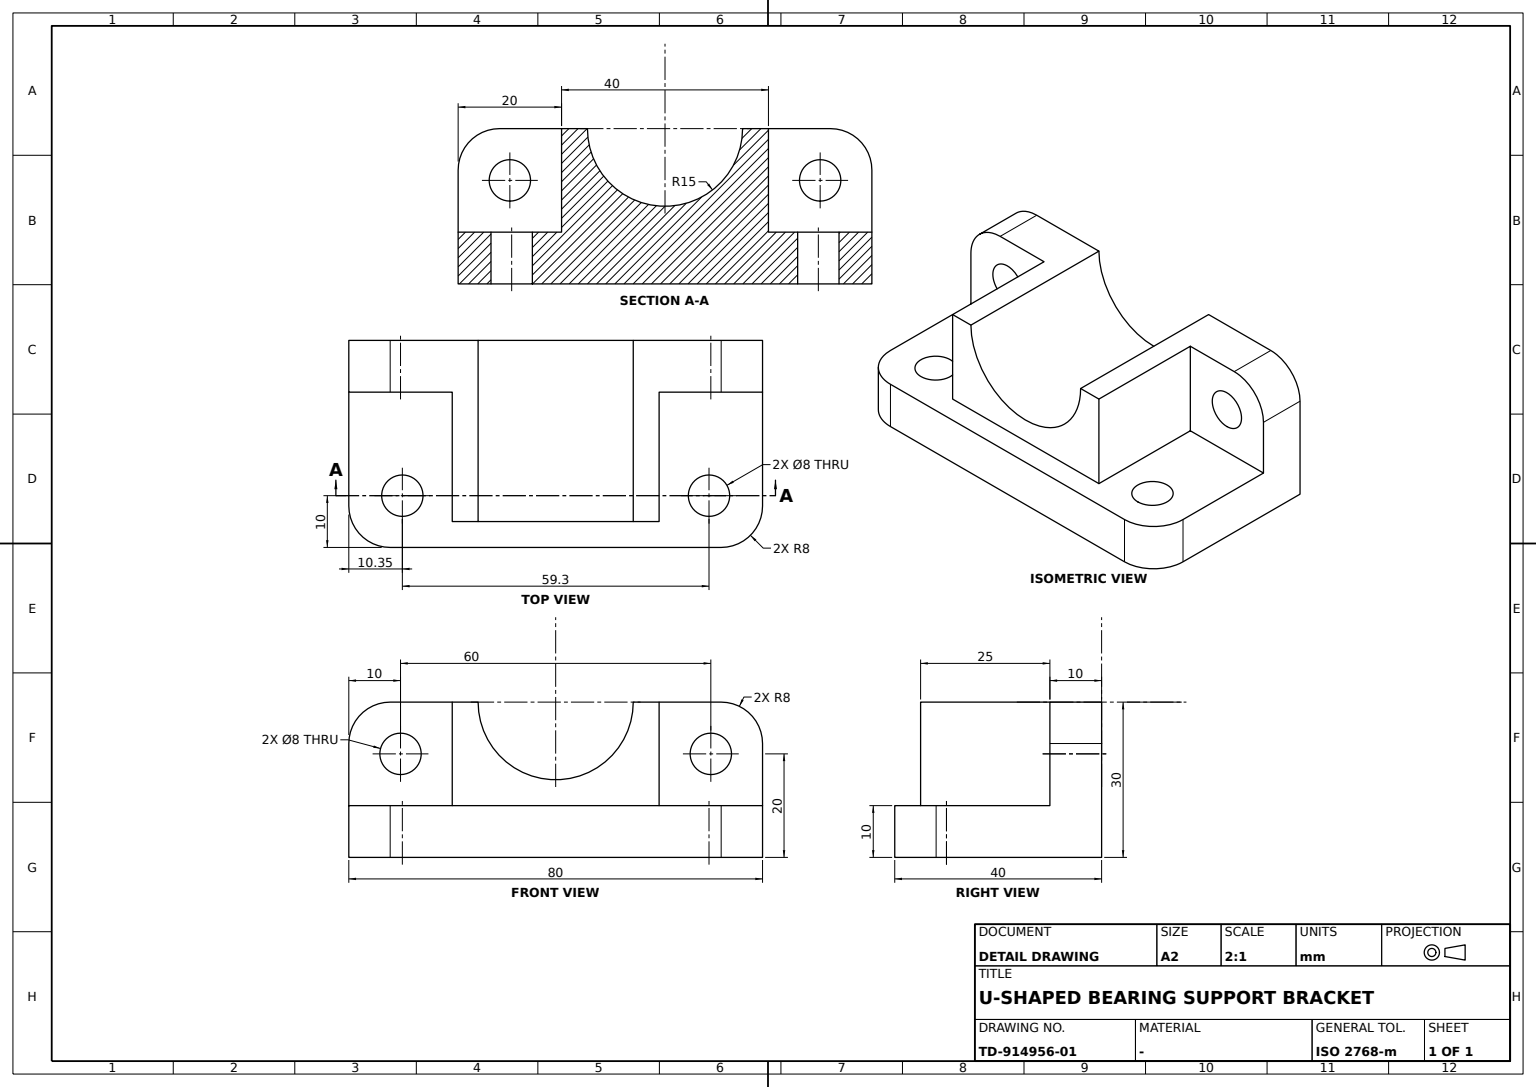
ISO-10303-21;
HEADER;
FILE_DESCRIPTION((''),'2;1');
FILE_NAME('','',(''),(''),'','','');
FILE_SCHEMA(('AUTOMOTIVE_DESIGN'));
ENDSEC;
DATA;
#1=APPLICATION_CONTEXT('');
#2=PRODUCT_CONTEXT('',#1,'mechanical');
#3=PRODUCT('','','',(#2));
#4=PRODUCT_DEFINITION_FORMATION('','',#3);
#5=PRODUCT_DEFINITION_CONTEXT('',#1,'design');
#6=PRODUCT_DEFINITION('','',#4,#5);
#7=PRODUCT_DEFINITION_SHAPE('','',#6);
#8=(LENGTH_UNIT()NAMED_UNIT(*)SI_UNIT(.MILLI.,.METRE.));
#9=(NAMED_UNIT(*)PLANE_ANGLE_UNIT()SI_UNIT($,.RADIAN.));
#10=(NAMED_UNIT(*)SI_UNIT($,.STERADIAN.)SOLID_ANGLE_UNIT());
#11=UNCERTAINTY_MEASURE_WITH_UNIT(LENGTH_MEASURE(0.005),#8,'distance_accuracy_value','');
#12=(GEOMETRIC_REPRESENTATION_CONTEXT(3)GLOBAL_UNCERTAINTY_ASSIGNED_CONTEXT((#11))GLOBAL_UNIT_ASSIGNED_CONTEXT((#8,#9,#10))REPRESENTATION_CONTEXT('',''));
#13=CARTESIAN_POINT('',(32.,-40.,-5.));
#14=VERTEX_POINT('',#13);
#15=CARTESIAN_POINT('',(32.,-40.,-15.));
#16=VERTEX_POINT('',#15);
#17=CARTESIAN_POINT('',(32.,-40.,-4.));
#18=DIRECTION('',(0.,0.,-1.));
#19=VECTOR('',#18,1000.);
#20=LINE('',#17,#19);
#21=EDGE_CURVE('',#14,#16,#20,.T.);
#22=ORIENTED_EDGE('',*,*,#21,.F.);
#23=CARTESIAN_POINT('',(10.,-40.,-5.));
#24=VERTEX_POINT('',#23);
#25=CARTESIAN_POINT('',(0.,-40.,-5.));
#26=DIRECTION('',(1.,0.,0.));
#27=VECTOR('',#26,1000.);
#28=LINE('',#25,#27);
#29=EDGE_CURVE('',#24,#14,#28,.T.);
#30=ORIENTED_EDGE('',*,*,#29,.F.);
#31=CARTESIAN_POINT('',(10.,-40.,7.));
#32=VERTEX_POINT('',#31);
#33=CARTESIAN_POINT('',(10.,-40.,0.));
#34=DIRECTION('',(0.,0.,1.));
#35=VECTOR('',#34,1000.);
#36=LINE('',#33,#35);
#37=EDGE_CURVE('',#24,#32,#36,.T.);
#38=ORIENTED_EDGE('',*,*,#37,.T.);
#39=CARTESIAN_POINT('',(0.,-40.,7.));
#40=VERTEX_POINT('',#39);
#41=CARTESIAN_POINT('',(5.,-40.,7.));
#42=LINE('',#41,#27);
#43=EDGE_CURVE('',#40,#32,#42,.T.);
#44=ORIENTED_EDGE('',*,*,#43,.F.);
#45=CARTESIAN_POINT('',(0.,-40.,-15.));
#46=VERTEX_POINT('',#45);
#47=CARTESIAN_POINT('',(0.,-40.,0.));
#48=LINE('',#47,#35);
#49=EDGE_CURVE('',#46,#40,#48,.T.);
#50=ORIENTED_EDGE('',*,*,#49,.F.);
#51=LINE('',#45,#27);
#52=EDGE_CURVE('',#46,#16,#51,.T.);
#53=ORIENTED_EDGE('',*,*,#52,.T.);
#54=EDGE_LOOP('',(#22,#30,#38,#44,#50,#53));
#55=FACE_BOUND('',#54,.T.);
#56=DIRECTION('',(0.,1.,0.));
#57=AXIS2_PLACEMENT_3D('',#45,#56,#34);
#58=PLANE('',#57);
#59=ADVANCED_FACE('',(#55),#58,.F.);
#60=CARTESIAN_POINT('',(0.,30.,1.));
#61=VERTEX_POINT('',#60);
#62=CARTESIAN_POINT('',(0.,30.,5.));
#63=AXIS2_PLACEMENT_3D('',#62,#26,#18);
#64=CIRCLE('',#63,4.);
#65=EDGE_CURVE('',#61,#61,#64,.T.);
#66=ORIENTED_EDGE('',*,*,#65,.T.);
#67=EDGE_LOOP('',(#66));
#68=FACE_BOUND('',#67,.T.);
#69=CARTESIAN_POINT('',(0.,-30.,1.));
#70=VERTEX_POINT('',#69);
#71=CARTESIAN_POINT('',(0.,-30.,5.));
#72=AXIS2_PLACEMENT_3D('',#71,#26,#18);
#73=CIRCLE('',#72,4.);
#74=EDGE_CURVE('',#70,#70,#73,.T.);
#75=ORIENTED_EDGE('',*,*,#74,.T.);
#76=EDGE_LOOP('',(#75));
#77=FACE_BOUND('',#76,.T.);
#78=CARTESIAN_POINT('',(0.,-15.,15.));
#79=VERTEX_POINT('',#78);
#80=CARTESIAN_POINT('',(0.,15.,15.));
#81=VERTEX_POINT('',#80);
#82=CARTESIAN_POINT('',(0.,0.,15.));
#83=AXIS2_PLACEMENT_3D('',#82,#26,#18);
#84=CIRCLE('',#83,15.);
#85=EDGE_CURVE('',#79,#81,#84,.T.);
#86=ORIENTED_EDGE('',*,*,#85,.T.);
#87=CARTESIAN_POINT('',(0.,32.,15.));
#88=VERTEX_POINT('',#87);
#89=VECTOR('',#56,1000.);
#90=LINE('',#82,#89);
#91=EDGE_CURVE('',#81,#88,#90,.T.);
#92=ORIENTED_EDGE('',*,*,#91,.T.);
#93=CARTESIAN_POINT('',(0.,40.,7.));
#94=VERTEX_POINT('',#93);
#95=CARTESIAN_POINT('',(0.,32.,7.));
#96=AXIS2_PLACEMENT_3D('',#95,#26,#18);
#97=CIRCLE('',#96,8.);
#98=EDGE_CURVE('',#94,#88,#97,.T.);
#99=ORIENTED_EDGE('',*,*,#98,.F.);
#100=CARTESIAN_POINT('',(0.,40.,-15.));
#101=VERTEX_POINT('',#100);
#102=CARTESIAN_POINT('',(0.,40.,0.));
#103=LINE('',#102,#19);
#104=EDGE_CURVE('',#94,#101,#103,.T.);
#105=ORIENTED_EDGE('',*,*,#104,.T.);
#106=CARTESIAN_POINT('',(0.,0.,-15.));
#107=DIRECTION('',(0.,-1.,0.));
#108=VECTOR('',#107,1000.);
#109=LINE('',#106,#108);
#110=EDGE_CURVE('',#101,#46,#109,.T.);
#111=ORIENTED_EDGE('',*,*,#110,.T.);
#112=ORIENTED_EDGE('',*,*,#49,.T.);
#113=CARTESIAN_POINT('',(0.,-32.,15.));
#114=VERTEX_POINT('',#113);
#115=CARTESIAN_POINT('',(0.,-32.,7.));
#116=AXIS2_PLACEMENT_3D('',#115,#26,#18);
#117=CIRCLE('',#116,8.);
#118=EDGE_CURVE('',#114,#40,#117,.T.);
#119=ORIENTED_EDGE('',*,*,#118,.F.);
#120=EDGE_CURVE('',#114,#79,#90,.T.);
#121=ORIENTED_EDGE('',*,*,#120,.T.);
#122=EDGE_LOOP('',(#86,#92,#99,#105,#111,#112,#119,#121));
#123=FACE_BOUND('',#122,.T.);
#124=CARTESIAN_POINT('',(0.,0.,0.));
#125=AXIS2_PLACEMENT_3D('',#124,#26,#56);
#126=PLANE('',#125);
#127=ADVANCED_FACE('',(#68,#77,#123),#126,.F.);
#128=CARTESIAN_POINT('',(40.,-32.,-15.));
#129=VERTEX_POINT('',#128);
#130=CARTESIAN_POINT('',(32.,-32.,-15.));
#131=AXIS2_PLACEMENT_3D('',#130,#34,#26);
#132=CIRCLE('',#131,8.);
#133=EDGE_CURVE('',#16,#129,#132,.T.);
#134=ORIENTED_EDGE('',*,*,#133,.T.);
#135=CARTESIAN_POINT('',(40.,-32.,-5.));
#136=VERTEX_POINT('',#135);
#137=CARTESIAN_POINT('',(40.,-32.,-4.));
#138=LINE('',#137,#19);
#139=EDGE_CURVE('',#136,#129,#138,.T.);
#140=ORIENTED_EDGE('',*,*,#139,.F.);
#141=CARTESIAN_POINT('',(32.,-32.,-5.));
#142=AXIS2_PLACEMENT_3D('',#141,#34,#26);
#143=CIRCLE('',#142,8.);
#144=EDGE_CURVE('',#14,#136,#143,.T.);
#145=ORIENTED_EDGE('',*,*,#144,.F.);
#146=ORIENTED_EDGE('',*,*,#21,.T.);
#147=EDGE_LOOP('',(#134,#140,#145,#146));
#148=FACE_BOUND('',#147,.T.);
#149=CARTESIAN_POINT('',(32.,-32.,-4.));
#150=AXIS2_PLACEMENT_3D('',#149,#18,#107);
#151=CYLINDRICAL_SURFACE('',#150,8.);
#152=ADVANCED_FACE('',(#148),#151,.T.);
#153=CARTESIAN_POINT('',(40.,32.,-15.));
#154=VERTEX_POINT('',#153);
#155=CARTESIAN_POINT('',(40.,32.,-5.));
#156=VERTEX_POINT('',#155);
#157=CARTESIAN_POINT('',(40.,32.,-4.));
#158=LINE('',#157,#35);
#159=EDGE_CURVE('',#154,#156,#158,.T.);
#160=ORIENTED_EDGE('',*,*,#159,.T.);
#161=CARTESIAN_POINT('',(40.,0.,-5.));
#162=LINE('',#161,#108);
#163=EDGE_CURVE('',#156,#136,#162,.T.);
#164=ORIENTED_EDGE('',*,*,#163,.T.);
#165=ORIENTED_EDGE('',*,*,#139,.T.);
#166=CARTESIAN_POINT('',(40.,40.,-15.));
#167=LINE('',#166,#89);
#168=EDGE_CURVE('',#129,#154,#167,.T.);
#169=ORIENTED_EDGE('',*,*,#168,.T.);
#170=EDGE_LOOP('',(#160,#164,#165,#169));
#171=FACE_BOUND('',#170,.T.);
#172=CARTESIAN_POINT('',(40.,0.,0.));
#173=AXIS2_PLACEMENT_3D('',#172,#26,#56);
#174=PLANE('',#173);
#175=ADVANCED_FACE('',(#171),#174,.T.);
#176=ORIENTED_EDGE('',*,*,#37,.F.);
#177=CARTESIAN_POINT('',(10.,-20.,-5.));
#178=VERTEX_POINT('',#177);
#179=CARTESIAN_POINT('',(10.,0.,-5.));
#180=LINE('',#179,#108);
#181=EDGE_CURVE('',#178,#24,#180,.T.);
#182=ORIENTED_EDGE('',*,*,#181,.F.);
#183=CARTESIAN_POINT('',(10.,-20.,15.));
#184=VERTEX_POINT('',#183);
#185=CARTESIAN_POINT('',(10.,-20.,0.));
#186=LINE('',#185,#19);
#187=EDGE_CURVE('',#184,#178,#186,.T.);
#188=ORIENTED_EDGE('',*,*,#187,.F.);
#189=CARTESIAN_POINT('',(10.,-32.,15.));
#190=VERTEX_POINT('',#189);
#191=CARTESIAN_POINT('',(10.,0.,15.));
#192=LINE('',#191,#89);
#193=EDGE_CURVE('',#190,#184,#192,.T.);
#194=ORIENTED_EDGE('',*,*,#193,.F.);
#195=CARTESIAN_POINT('',(10.,-32.,7.));
#196=AXIS2_PLACEMENT_3D('',#195,#26,#18);
#197=CIRCLE('',#196,8.);
#198=EDGE_CURVE('',#190,#32,#197,.T.);
#199=ORIENTED_EDGE('',*,*,#198,.T.);
#200=EDGE_LOOP('',(#176,#182,#188,#194,#199));
#201=FACE_BOUND('',#200,.T.);
#202=CARTESIAN_POINT('',(10.,-30.,1.));
#203=VERTEX_POINT('',#202);
#204=CARTESIAN_POINT('',(10.,-30.,5.));
#205=AXIS2_PLACEMENT_3D('',#204,#26,#18);
#206=CIRCLE('',#205,4.);
#207=EDGE_CURVE('',#203,#203,#206,.T.);
#208=ORIENTED_EDGE('',*,*,#207,.F.);
#209=EDGE_LOOP('',(#208));
#210=FACE_BOUND('',#209,.T.);
#211=CARTESIAN_POINT('',(10.,0.,0.));
#212=AXIS2_PLACEMENT_3D('',#211,#26,#56);
#213=PLANE('',#212);
#214=ADVANCED_FACE('',(#201,#210),#213,.T.);
#215=CARTESIAN_POINT('',(35.,15.,15.));
#216=VERTEX_POINT('',#215);
#217=CARTESIAN_POINT('',(35.,20.,15.));
#218=VERTEX_POINT('',#217);
#219=CARTESIAN_POINT('',(35.,0.,15.));
#220=LINE('',#219,#89);
#221=EDGE_CURVE('',#216,#218,#220,.T.);
#222=ORIENTED_EDGE('',*,*,#221,.F.);
#223=CARTESIAN_POINT('',(35.,-15.,15.));
#224=VERTEX_POINT('',#223);
#225=AXIS2_PLACEMENT_3D('',#219,#26,#18);
#226=CIRCLE('',#225,15.);
#227=EDGE_CURVE('',#224,#216,#226,.T.);
#228=ORIENTED_EDGE('',*,*,#227,.F.);
#229=CARTESIAN_POINT('',(35.,-20.,15.));
#230=VERTEX_POINT('',#229);
#231=EDGE_CURVE('',#230,#224,#220,.T.);
#232=ORIENTED_EDGE('',*,*,#231,.F.);
#233=CARTESIAN_POINT('',(35.,-20.,-5.));
#234=VERTEX_POINT('',#233);
#235=CARTESIAN_POINT('',(35.,-20.,0.));
#236=LINE('',#235,#19);
#237=EDGE_CURVE('',#230,#234,#236,.T.);
#238=ORIENTED_EDGE('',*,*,#237,.T.);
#239=CARTESIAN_POINT('',(35.,20.,-5.));
#240=VERTEX_POINT('',#239);
#241=CARTESIAN_POINT('',(35.,0.,-5.));
#242=LINE('',#241,#108);
#243=EDGE_CURVE('',#240,#234,#242,.T.);
#244=ORIENTED_EDGE('',*,*,#243,.F.);
#245=CARTESIAN_POINT('',(35.,20.,0.));
#246=LINE('',#245,#19);
#247=EDGE_CURVE('',#218,#240,#246,.T.);
#248=ORIENTED_EDGE('',*,*,#247,.F.);
#249=EDGE_LOOP('',(#222,#228,#232,#238,#244,#248));
#250=FACE_BOUND('',#249,.T.);
#251=CARTESIAN_POINT('',(35.,0.,0.));
#252=AXIS2_PLACEMENT_3D('',#251,#26,#56);
#253=PLANE('',#252);
#254=ADVANCED_FACE('',(#250),#253,.T.);
#255=ORIENTED_EDGE('',*,*,#104,.F.);
#256=CARTESIAN_POINT('',(10.,40.,7.));
#257=VERTEX_POINT('',#256);
#258=CARTESIAN_POINT('',(5.,40.,7.));
#259=LINE('',#258,#27);
#260=EDGE_CURVE('',#94,#257,#259,.T.);
#261=ORIENTED_EDGE('',*,*,#260,.T.);
#262=CARTESIAN_POINT('',(10.,40.,-5.));
#263=VERTEX_POINT('',#262);
#264=CARTESIAN_POINT('',(10.,40.,0.));
#265=LINE('',#264,#19);
#266=EDGE_CURVE('',#257,#263,#265,.T.);
#267=ORIENTED_EDGE('',*,*,#266,.T.);
#268=CARTESIAN_POINT('',(32.,40.,-5.));
#269=VERTEX_POINT('',#268);
#270=LINE('',#262,#27);
#271=EDGE_CURVE('',#263,#269,#270,.T.);
#272=ORIENTED_EDGE('',*,*,#271,.T.);
#273=CARTESIAN_POINT('',(32.,40.,-15.));
#274=VERTEX_POINT('',#273);
#275=CARTESIAN_POINT('',(32.,40.,-4.));
#276=LINE('',#275,#35);
#277=EDGE_CURVE('',#274,#269,#276,.T.);
#278=ORIENTED_EDGE('',*,*,#277,.F.);
#279=LINE('',#100,#27);
#280=EDGE_CURVE('',#101,#274,#279,.T.);
#281=ORIENTED_EDGE('',*,*,#280,.F.);
#282=EDGE_LOOP('',(#255,#261,#267,#272,#278,#281));
#283=FACE_BOUND('',#282,.T.);
#284=CARTESIAN_POINT('',(0.,40.,15.));
#285=AXIS2_PLACEMENT_3D('',#284,#107,#18);
#286=PLANE('',#285);
#287=ADVANCED_FACE('',(#283),#286,.F.);
#288=CARTESIAN_POINT('',(34.,29.648144,-15.));
#289=VERTEX_POINT('',#288);
#290=CARTESIAN_POINT('',(30.,29.648144,-15.));
#291=AXIS2_PLACEMENT_3D('',#290,#34,#26);
#292=CIRCLE('',#291,4.);
#293=EDGE_CURVE('',#289,#289,#292,.T.);
#294=ORIENTED_EDGE('',*,*,#293,.F.);
#295=EDGE_LOOP('',(#294));
#296=FACE_BOUND('',#295,.T.);
#297=CARTESIAN_POINT('',(34.,29.648144,-5.));
#298=VERTEX_POINT('',#297);
#299=CARTESIAN_POINT('',(30.,29.648144,-5.));
#300=AXIS2_PLACEMENT_3D('',#299,#34,#26);
#301=CIRCLE('',#300,4.);
#302=EDGE_CURVE('',#298,#298,#301,.T.);
#303=ORIENTED_EDGE('',*,*,#302,.T.);
#304=EDGE_LOOP('',(#303));
#305=FACE_BOUND('',#304,.T.);
#306=CARTESIAN_POINT('',(30.,29.648144,-10.66));
#307=AXIS2_PLACEMENT_3D('',#306,#34,#26);
#308=CYLINDRICAL_SURFACE('',#307,4.);
#309=ADVANCED_FACE('',(#296,#305),#308,.F.);
#310=LINE('',#223,#27);
#311=EDGE_CURVE('',#224,#79,#310,.F.);
#312=ORIENTED_EDGE('',*,*,#311,.T.);
#313=ORIENTED_EDGE('',*,*,#120,.F.);
#314=CARTESIAN_POINT('',(5.,-32.,15.));
#315=LINE('',#314,#27);
#316=EDGE_CURVE('',#114,#190,#315,.T.);
#317=ORIENTED_EDGE('',*,*,#316,.T.);
#318=ORIENTED_EDGE('',*,*,#193,.T.);
#319=LINE('',#183,#27);
#320=EDGE_CURVE('',#184,#230,#319,.T.);
#321=ORIENTED_EDGE('',*,*,#320,.T.);
#322=ORIENTED_EDGE('',*,*,#231,.T.);
#323=EDGE_LOOP('',(#312,#313,#317,#318,#321,#322));
#324=FACE_BOUND('',#323,.T.);
#325=CARTESIAN_POINT('',(0.,-40.,15.));
#326=AXIS2_PLACEMENT_3D('',#325,#18,#56);
#327=PLANE('',#326);
#328=ADVANCED_FACE('',(#324),#327,.F.);
#329=ORIENTED_EDGE('',*,*,#98,.T.);
#330=CARTESIAN_POINT('',(10.,32.,15.));
#331=VERTEX_POINT('',#330);
#332=CARTESIAN_POINT('',(5.,32.,15.));
#333=LINE('',#332,#27);
#334=EDGE_CURVE('',#88,#331,#333,.T.);
#335=ORIENTED_EDGE('',*,*,#334,.T.);
#336=CARTESIAN_POINT('',(10.,32.,7.));
#337=AXIS2_PLACEMENT_3D('',#336,#26,#18);
#338=CIRCLE('',#337,8.);
#339=EDGE_CURVE('',#257,#331,#338,.T.);
#340=ORIENTED_EDGE('',*,*,#339,.F.);
#341=ORIENTED_EDGE('',*,*,#260,.F.);
#342=EDGE_LOOP('',(#329,#335,#340,#341));
#343=FACE_BOUND('',#342,.T.);
#344=CARTESIAN_POINT('',(5.,32.,7.));
#345=AXIS2_PLACEMENT_3D('',#344,#26,#34);
#346=CYLINDRICAL_SURFACE('',#345,8.);
#347=ADVANCED_FACE('',(#343),#346,.T.);
#348=CARTESIAN_POINT('',(34.,-29.648144,-15.));
#349=VERTEX_POINT('',#348);
#350=CARTESIAN_POINT('',(30.,-29.648144,-15.));
#351=AXIS2_PLACEMENT_3D('',#350,#34,#26);
#352=CIRCLE('',#351,4.);
#353=EDGE_CURVE('',#349,#349,#352,.T.);
#354=ORIENTED_EDGE('',*,*,#353,.F.);
#355=EDGE_LOOP('',(#354));
#356=FACE_BOUND('',#355,.T.);
#357=CARTESIAN_POINT('',(34.,-29.648144,-5.));
#358=VERTEX_POINT('',#357);
#359=CARTESIAN_POINT('',(30.,-29.648144,-5.));
#360=AXIS2_PLACEMENT_3D('',#359,#34,#26);
#361=CIRCLE('',#360,4.);
#362=EDGE_CURVE('',#358,#358,#361,.T.);
#363=ORIENTED_EDGE('',*,*,#362,.T.);
#364=EDGE_LOOP('',(#363));
#365=FACE_BOUND('',#364,.T.);
#366=CARTESIAN_POINT('',(30.,-29.648144,-10.66));
#367=AXIS2_PLACEMENT_3D('',#366,#34,#26);
#368=CYLINDRICAL_SURFACE('',#367,4.);
#369=ADVANCED_FACE('',(#356,#365),#368,.F.);
#370=ORIENTED_EDGE('',*,*,#362,.F.);
#371=EDGE_LOOP('',(#370));
#372=FACE_BOUND('',#371,.T.);
#373=ORIENTED_EDGE('',*,*,#243,.T.);
#374=LINE('',#177,#27);
#375=EDGE_CURVE('',#178,#234,#374,.T.);
#376=ORIENTED_EDGE('',*,*,#375,.F.);
#377=ORIENTED_EDGE('',*,*,#181,.T.);
#378=ORIENTED_EDGE('',*,*,#29,.T.);
#379=ORIENTED_EDGE('',*,*,#144,.T.);
#380=ORIENTED_EDGE('',*,*,#163,.F.);
#381=CARTESIAN_POINT('',(32.,32.,-5.));
#382=AXIS2_PLACEMENT_3D('',#381,#34,#26);
#383=CIRCLE('',#382,8.);
#384=EDGE_CURVE('',#156,#269,#383,.T.);
#385=ORIENTED_EDGE('',*,*,#384,.T.);
#386=ORIENTED_EDGE('',*,*,#271,.F.);
#387=CARTESIAN_POINT('',(10.,20.,-5.));
#388=VERTEX_POINT('',#387);
#389=EDGE_CURVE('',#263,#388,#180,.T.);
#390=ORIENTED_EDGE('',*,*,#389,.T.);
#391=LINE('',#387,#27);
#392=EDGE_CURVE('',#388,#240,#391,.T.);
#393=ORIENTED_EDGE('',*,*,#392,.T.);
#394=EDGE_LOOP('',(#373,#376,#377,#378,#379,#380,#385,#386,#390,#393));
#395=FACE_BOUND('',#394,.T.);
#396=ORIENTED_EDGE('',*,*,#302,.F.);
#397=EDGE_LOOP('',(#396));
#398=FACE_BOUND('',#397,.T.);
#399=AXIS2_PLACEMENT_3D('',#262,#34,#107);
#400=PLANE('',#399);
#401=ADVANCED_FACE('',(#372,#395,#398),#400,.T.);
#402=LINE('',#215,#27);
#403=EDGE_CURVE('',#81,#216,#402,.T.);
#404=ORIENTED_EDGE('',*,*,#403,.F.);
#405=ORIENTED_EDGE('',*,*,#85,.F.);
#406=ORIENTED_EDGE('',*,*,#311,.F.);
#407=ORIENTED_EDGE('',*,*,#227,.T.);
#408=EDGE_LOOP('',(#404,#405,#406,#407));
#409=FACE_BOUND('',#408,.T.);
#410=CARTESIAN_POINT('',(16.84,0.,15.));
#411=AXIS2_PLACEMENT_3D('',#410,#26,#56);
#412=CYLINDRICAL_SURFACE('',#411,15.);
#413=ADVANCED_FACE('',(#409),#412,.F.);
#414=ORIENTED_EDGE('',*,*,#207,.T.);
#415=EDGE_LOOP('',(#414));
#416=FACE_BOUND('',#415,.T.);
#417=ORIENTED_EDGE('',*,*,#74,.F.);
#418=EDGE_LOOP('',(#417));
#419=FACE_BOUND('',#418,.T.);
#420=CARTESIAN_POINT('',(5.,-30.,5.));
#421=AXIS2_PLACEMENT_3D('',#420,#26,#56);
#422=CYLINDRICAL_SURFACE('',#421,4.);
#423=ADVANCED_FACE('',(#416,#419),#422,.F.);
#424=ORIENTED_EDGE('',*,*,#65,.F.);
#425=EDGE_LOOP('',(#424));
#426=FACE_BOUND('',#425,.T.);
#427=CARTESIAN_POINT('',(10.,30.,1.));
#428=VERTEX_POINT('',#427);
#429=CARTESIAN_POINT('',(10.,30.,5.));
#430=AXIS2_PLACEMENT_3D('',#429,#26,#18);
#431=CIRCLE('',#430,4.);
#432=EDGE_CURVE('',#428,#428,#431,.T.);
#433=ORIENTED_EDGE('',*,*,#432,.T.);
#434=EDGE_LOOP('',(#433));
#435=FACE_BOUND('',#434,.T.);
#436=CARTESIAN_POINT('',(5.,30.,5.));
#437=AXIS2_PLACEMENT_3D('',#436,#26,#56);
#438=CYLINDRICAL_SURFACE('',#437,4.);
#439=ADVANCED_FACE('',(#426,#435),#438,.F.);
#440=CARTESIAN_POINT('',(32.,32.,-15.));
#441=AXIS2_PLACEMENT_3D('',#440,#34,#26);
#442=CIRCLE('',#441,8.);
#443=EDGE_CURVE('',#154,#274,#442,.T.);
#444=ORIENTED_EDGE('',*,*,#443,.T.);
#445=ORIENTED_EDGE('',*,*,#277,.T.);
#446=ORIENTED_EDGE('',*,*,#384,.F.);
#447=ORIENTED_EDGE('',*,*,#159,.F.);
#448=EDGE_LOOP('',(#444,#445,#446,#447));
#449=FACE_BOUND('',#448,.T.);
#450=CARTESIAN_POINT('',(32.,32.,-4.));
#451=AXIS2_PLACEMENT_3D('',#450,#34,#56);
#452=CYLINDRICAL_SURFACE('',#451,8.);
#453=ADVANCED_FACE('',(#449),#452,.T.);
#454=ORIENTED_EDGE('',*,*,#353,.T.);
#455=EDGE_LOOP('',(#454));
#456=FACE_BOUND('',#455,.T.);
#457=ORIENTED_EDGE('',*,*,#443,.F.);
#458=ORIENTED_EDGE('',*,*,#168,.F.);
#459=ORIENTED_EDGE('',*,*,#133,.F.);
#460=ORIENTED_EDGE('',*,*,#52,.F.);
#461=ORIENTED_EDGE('',*,*,#110,.F.);
#462=ORIENTED_EDGE('',*,*,#280,.T.);
#463=EDGE_LOOP('',(#457,#458,#459,#460,#461,#462));
#464=FACE_BOUND('',#463,.T.);
#465=ORIENTED_EDGE('',*,*,#293,.T.);
#466=EDGE_LOOP('',(#465));
#467=FACE_BOUND('',#466,.T.);
#468=AXIS2_PLACEMENT_3D('',#100,#34,#107);
#469=PLANE('',#468);
#470=ADVANCED_FACE('',(#456,#464,#467),#469,.F.);
#471=CARTESIAN_POINT('',(10.,20.,15.));
#472=VERTEX_POINT('',#471);
#473=CARTESIAN_POINT('',(10.,20.,0.));
#474=LINE('',#473,#19);
#475=EDGE_CURVE('',#472,#388,#474,.T.);
#476=ORIENTED_EDGE('',*,*,#475,.F.);
#477=LINE('',#471,#27);
#478=EDGE_CURVE('',#472,#218,#477,.T.);
#479=ORIENTED_EDGE('',*,*,#478,.T.);
#480=ORIENTED_EDGE('',*,*,#247,.T.);
#481=ORIENTED_EDGE('',*,*,#392,.F.);
#482=EDGE_LOOP('',(#476,#479,#480,#481));
#483=FACE_BOUND('',#482,.T.);
#484=AXIS2_PLACEMENT_3D('',#471,#107,#18);
#485=PLANE('',#484);
#486=ADVANCED_FACE('',(#483),#485,.F.);
#487=ORIENTED_EDGE('',*,*,#432,.F.);
#488=EDGE_LOOP('',(#487));
#489=FACE_BOUND('',#488,.T.);
#490=ORIENTED_EDGE('',*,*,#339,.T.);
#491=EDGE_CURVE('',#472,#331,#192,.T.);
#492=ORIENTED_EDGE('',*,*,#491,.F.);
#493=ORIENTED_EDGE('',*,*,#475,.T.);
#494=ORIENTED_EDGE('',*,*,#389,.F.);
#495=ORIENTED_EDGE('',*,*,#266,.F.);
#496=EDGE_LOOP('',(#490,#492,#493,#494,#495));
#497=FACE_BOUND('',#496,.T.);
#498=ADVANCED_FACE('',(#489,#497),#213,.T.);
#499=ORIENTED_EDGE('',*,*,#198,.F.);
#500=ORIENTED_EDGE('',*,*,#316,.F.);
#501=ORIENTED_EDGE('',*,*,#118,.T.);
#502=ORIENTED_EDGE('',*,*,#43,.T.);
#503=EDGE_LOOP('',(#499,#500,#501,#502));
#504=FACE_BOUND('',#503,.T.);
#505=CARTESIAN_POINT('',(5.,-32.,7.));
#506=AXIS2_PLACEMENT_3D('',#505,#26,#107);
#507=CYLINDRICAL_SURFACE('',#506,8.);
#508=ADVANCED_FACE('',(#504),#507,.T.);
#509=ORIENTED_EDGE('',*,*,#91,.F.);
#510=ORIENTED_EDGE('',*,*,#403,.T.);
#511=ORIENTED_EDGE('',*,*,#221,.T.);
#512=ORIENTED_EDGE('',*,*,#478,.F.);
#513=ORIENTED_EDGE('',*,*,#491,.T.);
#514=ORIENTED_EDGE('',*,*,#334,.F.);
#515=EDGE_LOOP('',(#509,#510,#511,#512,#513,#514));
#516=FACE_BOUND('',#515,.T.);
#517=ADVANCED_FACE('',(#516),#327,.F.);
#518=ORIENTED_EDGE('',*,*,#237,.F.);
#519=ORIENTED_EDGE('',*,*,#320,.F.);
#520=ORIENTED_EDGE('',*,*,#187,.T.);
#521=ORIENTED_EDGE('',*,*,#375,.T.);
#522=EDGE_LOOP('',(#518,#519,#520,#521));
#523=FACE_BOUND('',#522,.T.);
#524=AXIS2_PLACEMENT_3D('',#183,#107,#18);
#525=PLANE('',#524);
#526=ADVANCED_FACE('',(#523),#525,.T.);
#527=CLOSED_SHELL('',(#59,#127,#152,#175,#214,#254,#287,#309,#328,#347,#369,#401,#413,#423,#439,#453,#470,#486,#498,#508,#517,#526));
#528=MANIFOLD_SOLID_BREP('',#527);
#529=ADVANCED_BREP_SHAPE_REPRESENTATION('',(#528),#12);
#530=SHAPE_DEFINITION_REPRESENTATION(#7,#529);
ENDSEC;
END-ISO-10303-21;
